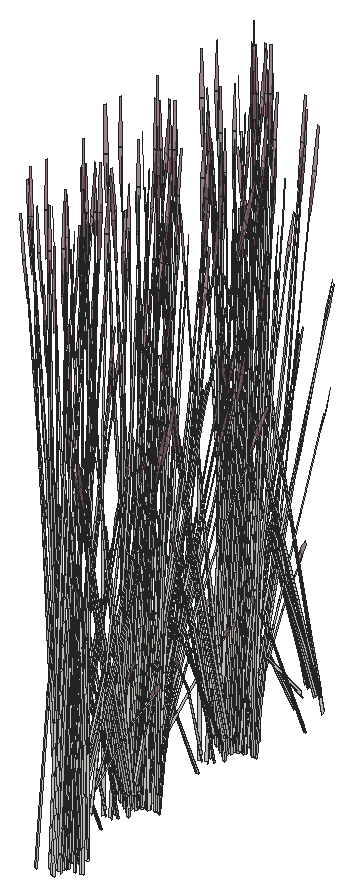
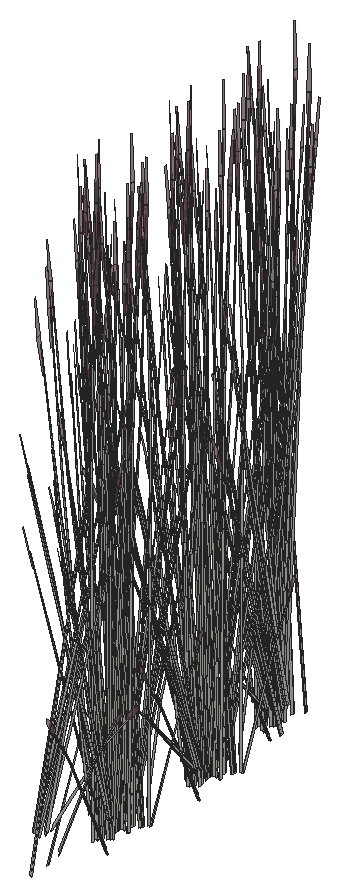
# SketchUp Ruby script. Lengths in inches.
U = 1.inch
M = Sketchup.active_model
def pt(a) = Geom::Point3d.new(a.map { |v| v * U })
def face(e, loops, mat)
  f = e.add_face(loops[0].map { |a| pt(a) })
  loops[1..].each { |l| e.add_face(l.map { |a| pt(a) }).erase! }
  f.material = f.back_material = mat if mat
  f
end
# faces: each face lists its corners as indices into pts; further lists are holes
def faces(e, pts, list, mat = nil) = list.each { |f| face(e, (f[0].is_a?(Array) ? f : [f]).map { |l| l.map { |i| pts[i] } }, mat) }
# xy, xz, yz: faces in a plane at the given z, y or x. An outline is a flat list of corners, or four numbers for a rectangle; further outlines are holes
def ring(l) = l.size == 4 ? [[l[0], l[1]], [l[2], l[1]], [l[2], l[3]], [l[0], l[3]]] : l.each_slice(2).to_a
def flat(e, list, mat, &to3) = list.each { |f| face(e, (f[0].is_a?(Array) ? f : [f]).map { |l| ring(l).map { |u, v| to3.(u, v) } }, mat) }
def xy(e, z, list, mat = nil) = flat(e, list, mat) { |x, y| [x, y, z] }
def xz(e, y, list, mat = nil) = flat(e, list, mat) { |x, z| [x, y, z] }
def yz(e, x, list, mat = nil) = flat(e, list, mat) { |y, z| [x, y, z] }
def lines(e, pts, list) = list.each { |a, b| e.add_line(pt(pts[a]), pt(pts[b])) }
# prism: a flat outline (further loops are holes) pulled along v
def prism(e, loops, v, mat = nil)
  f = face(e, loops, mat); d = Geom::Vector3d.new(v.map { |x| x * U })
  f.pushpull(f.normal.samedirection?(d) ? d.length : -d.length)
end
def box(e, o, s, mat = nil) = prism(e, [[o, [o[0] + s[0], o[1], o[2]], [o[0] + s[0], o[1] + s[1], o[2]], [o[0], o[1] + s[1], o[2]]]], [0, 0, s[2]], mat)
def at(x, y, z, deg = 0) = Geom::Transformation.translation(pt([x, y, z])) * Geom::Transformation.rotation(ORIGIN, Z_AXIS, deg.degrees)
def axes(o, x, y, z) = Geom::Transformation.new([*x, 0, *y, 0, *z, 0, *pt(o).to_a, 1])
def part(name) = M.definitions.add(name)
# library, detail: a bought-in or finely detailed component or shape, given as its bounding box
def library(name, o, s) = part(name).tap { |d| box(d.entities, o, s) }
def detail(e, o, s) = box(e.add_group.entities, o, s)
def put(e, d, t, mat = nil) = e.add_instance(d, t).tap { |i| i.material = mat if mat }
def group(e, t, mat = nil) = e.add_group.tap { |g| g.transformation = t; g.material = mat if mat }.entities
root = M.entities
M.materials.add("LightPink_Translucent").color = [144, 107, 117]
M.materials["LightPink_Translucent"].alpha = 0.75
c1 = part("blade")
p = [[2.15,0.21,22],[0,0.17,0],[0.09,0.45,0],[2.18,0.31,22],[2.29,0.31,22],[0.38,0.45,0],
  [2.48,0.24,33],[2.49,0.24,33],[2.48,0.22,33]]
faces(c1.entities,p,[[0,1,2,3],[4,5,2,3],[6,3,4,7],[8,0,3,6]])
c2 = part("seeds")
p = [[0.3,-0.1,1.38],[-0.01,-0.03,1.59],[-0.01,-0.03,0.03],[0.14,-0.07,-0.07],[0.29,-0.03,3],[0.15,0.01,3.11]]
faces(c2.entities,p,[[0,1,2,3],[1,0,4,5]],"LightPink_Translucent")
c3 = part("blade with seeds")
put(c3.entities,c1,at(0,0,0))
put(c3.entities,c2,axes([2.4,0.25,30.99],[1.5799,-0.05474,1.17369],[-0.12525,1.92788,0.29478],[-0.07173,-0.02425,1.56792]))
put(root,c3,axes([405.15,364.68,-9.95],[0,-0.62892,0],[0.63949,0,0],[0,0,1.6711]))
put(root,c3,axes([404.84,364.29,-9.8],[-0.42403,0.49328,0.42607],[-0.50377,-0.43543,0.16719],[0.10223,-0.04923,1.47927]))
put(root,c3,axes([405.31,365.17,-9.86],[-0.47569,-0.46784,-0.05709],[0.47598,-0.46812,0],[-0.01661,-0.01634,1.63492]))
put(root,c3,axes([404.11,363.47,-9.7],[-0.14774,0.54019,0.16428],[-0.54062,-0.15287,0.32672],[0.09339,-0.00263,1.49371]))
put(root,c3,axes([404.4,365.23,-9.8],[0.64638,0.11452,0.42607],[-0.13155,0.64678,0.16719],[-0.09446,-0.06245,1.47927]))
put(root,c3,axes([404.05,366.26,-9.7],[0.54955,-0.14427,0.16428],[0.1357,0.53689,0.32672],[-0.04901,-0.07823,1.49371]))
put(root,c3,axes([405.74,363.5,-9.7],[-0.54955,0.14427,0.16428],[-0.1357,-0.53689,0.32672],[0.04901,0.07823,1.49371]))
put(root,c3,axes([405.4,364.54,-9.78],[-0.64638,-0.11452,0.45814],[0.13155,-0.64678,0.17978],[0.09446,0.06245,1.59061]))
put(root,c3,axes([404.88,366.13,-9.95],[-0.16686,-0.46861,0],[0.47648,-0.16411,0],[0,0,1.4375]))
put(root,c3,axes([405.69,366.29,-9.7],[0.14774,-0.54019,0.16428],[0.54062,0.15287,0.32672],[-0.09339,0.00263,1.49371]))
put(root,c3,axes([405.57,365.0625,-9.9375],[0.35699,0.35109,0],[-0.35699,0.35109,0],[0,0,1.57621]))
put(root,c3,axes([406.53,364.91,-9.7],[-0.40181,-0.39593,0.16428],[0.40492,-0.38402,0.32672],[-0.04438,0.08086,1.49371]))
put(root,c3,axes([404.76,366.34,-9.95],[-0.51557,-0.24403,0],[0.24813,-0.50705,0],[0,0,1.51513]))
put(root,c3,axes([405.5625,364.65,-9.47],[0.24813,-0.48978,0.41661],[0.51557,0.23571,-0.2005],[0,0.1129,1.33761]))
put(root,c3,axes([405.47,364.93,-9.87],[0,0.62861,-0.05249],[-0.63949,0,0],[0,0.01975,1.67027]))
put(root,c3,axes([405.43,365.33,-9.47],[0.55535,-0.03355,0.41661],[0.05022,0.55698,-0.2005],[-0.09942,0.05645,1.33761]))
put(root,c3,axes([405.35,366.35,-9.95],[0.51557,0.24403,0],[-0.24813,0.50705,0],[0,0,1.62917]))
put(root,c3,axes([405.55,366.89,-9.96],[-0.31576,-0.54657,-0.04789],[0.53494,-0.30375,0.48057],[-0.13182,0.05204,1.52373]))
put(root,c3,axes([405.44,365.57,-9.5625],[0.37783,0.32657,0.13483],[-0.31516,0.36844,-0.38503],[-0.08772,0.04981,1.18024]))
put(root,c3,axes([405.84,366.58,-9.69],[0.47863,-0.27177,0.46235],[0.28609,0.48733,0],[-0.10901,0.0619,1.46668]))
put(root,c3,axes([405.16,366.15,-9.87],[0.22235,0.62444,-0.05599],[-0.63531,0.21881,0],[0.00776,0.02181,1.60327]))
put(root,c3,axes([405.41,366.82,-10.11],[-0.47712,-0.13449,-0.28847],[0.12013,-0.47362,0.28847],[-0.09619,0.05462,1.29413]))
put(root,c3,axes([407,365.33,-9.95],[-0.63917,-0.00435,-0.04634],[0,-0.60749,0.46507],[-0.02009,0.13829,1.47457]))
put(root,c3,axes([405.33,365.45,-9.52],[0.05959,0.62022,-0.27094],[-0.62068,0.0375,-0.46562],[-0.1093,0.08261,1.4872]))
put(root,c3,axes([405.55,365.21,-9.94],[-0.24813,0.48978,-0.41661],[-0.51557,-0.23571,0.2005],[0,0.1129,1.33761]))
put(root,c3,axes([405.57,366.61,-9.83],[0.64025,0.17667,0.2864],[-0.16018,0.63149,-0.33981],[-0.10597,0.07904,1.53541]))
put(root,c3,axes([405.52,367.04,-10.12],[-0.47863,0.27177,-0.46235],[-0.28609,-0.48733,0],[-0.10901,0.0619,1.46668]))
put(root,c3,axes([404.15,373.01,-9.59],[-0.14537,0.11002,1.33163],[-0.43536,-0.19256,-0.28638],[0.0807,-0.23948,0.56934]))
put(root,c3,axes([403.36,366.375,-7.3],[0.34603,-0.28618,0.32977],[0.32756,0.32677,-0.42575],[-0.04984,0.16603,0.81462]))
put(root,c3,axes([405.95,366.96,-9.79],[0.31974,0.54466,0],[-0.53494,0.30375,-0.48057],[-0.12184,0.06918,1.52448]))
put(root,c3,axes([403.07,372.41,-10.61],[-0.08578,0.01958,1.6421],[-0.47437,-0.22044,-0.25086],[0.00796,-0.18387,0.2797]))
put(root,c3,axes([405.68,364.8,-9.35],[-0.01397,-0.51177,1.31553],[0.63227,0.13266,0.557],[-0.14954,0.28003,1.24175]))
put(root,c3,axes([404.5,373.82,-7.36],[0.01331,-0.50278,-0.66157],[0.56035,0.03377,0.07984],[0.05914,-0.213,0.93586]))
put(root,c3,axes([404.33,366.85,-7.3],[0.15418,-0.41799,0.32977],[0.44981,0.12192,-0.42575],[0.04124,0.16829,0.81462]))
put(root,c3,axes([403.53,373.02,-7.78],[0.15418,-0.41799,-0.32977],[0.44981,0.12192,0.42575],[-0.04124,-0.16829,0.81462]))
put(root,c3,axes([405.17,372.65,-7.62],[-0.05194,0.04152,1.65179],[-0.50886,-0.14007,-0.15608],[-0.01842,-0.18118,0.29231]))
put(root,c3,axes([403.62,372.13,-9.42],[0.06561,0.31695,1.06958],[-0.36394,-0.17555,0.78586],[0.03916,-0.16229,0.23558]))
put(root,c3,axes([404.39,373.66,-7.64],[-0.3661,-0.36521,-0.47583],[0.38674,-0.31985,-0.36857],[0.0557,-0.18556,0.91046]))
put(root,c3,axes([404.9375,368.34,-6.74],[0.35341,-0.31182,-0.06041],[0.32382,0.34152,-0.27392],[0.0228,0.09677,0.90349]))
put(root,c3,axes([403.59,373.11,-7.59],[0.50393,0.1421,0.447],[-0.17232,0.46717,0.36857],[-0.03028,-0.18372,0.92496]))
put(root,c3,axes([404.19,367.23,-7.6],[-0.37684,0.18473,0.05988],[-0.18445,-0.33686,0.47138],[0.03639,0.14849,0.71878]))
put(root,c3,axes([404.77,373.85,-7.3125],[-0.56206,-0.02693,-0.11324],[0.01536,-0.50991,-0.62851],[0.03904,-0.19638,0.95501]))
put(root,c3,axes([403.14,366.45,-6.97],[0.56206,0.02693,-0.12569],[-0.01536,0.50991,-0.69765],[-0.03904,0.19638,1.06006]))
put(root,c3,axes([404.73,373.52,-7.78],[0.34603,-0.28618,-0.32977],[0.32756,0.32677,0.42575],[0.04984,-0.16603,0.81462]))
put(root,c3,axes([404.18,367.02,-7.3125],[0.50045,-0.25306,-0.11324],[0.24593,0.44915,-0.62851],[0.06603,0.18927,0.95501]))
put(root,c3,axes([403.72,373.08,-7.6],[0.37684,-0.18473,0.05988],[0.18445,0.33686,0.47138],[-0.03639,-0.14849,0.71878]))
put(root,c3,axes([404.33,367.19,-7.28],[-0.50393,-0.1421,0.49617],[0.17232,-0.46717,0.40911],[0.03028,0.18372,1.0267]))
put(root,c3,axes([404.27,367.12,-10.61],[0.08277,-0.02958,1.6421],[0.49786,0.16279,-0.25086],[0.01456,0.18348,0.2797]))
put(root,c3,axes([403.53,366.65,-7.34],[0.3661,0.36521,-0.52818],[-0.38674,0.31985,-0.40911],[-0.0557,0.18556,1.01061]))
put(root,c3,axes([403.13,367.2,-9.37],[0.46459,-0.09625,0.0606],[0.10681,0.38778,-0.80367],[-0.02945,0.1963,0.72038]))
put(root,c3,axes([404.61,367,-7.64],[0.50273,0.13626,-0.47583],[-0.17232,0.46717,-0.36857],[0.0461,0.18809,0.91046]))
put(root,c3,axes([404.38,367.29,-7.78],[-0.15418,0.41799,-0.32977],[-0.44981,-0.12192,0.42575],[0.04124,0.16829,0.81462]))
put(root,c3,axes([403.94,366.12,-8.39],[-0.01252,-0.20862,1.59586],[0.54251,0.1384,0.12904],[-0.03356,0.2973,0.68222]))
put(root,c3,axes([404.55,373.93,-7.3],[-0.34603,0.28618,0.32977],[-0.32756,-0.32677,-0.42575],[0.04984,-0.16603,0.81462]))
put(root,c3,axes([402.28,373.45,-9.79],[-0.31974,-0.54466,0],[0.53494,-0.30375,-0.48057],[0.12184,-0.06918,1.52448]))
put(root,c3,axes([404.43,366.91,-7.36],[0.24409,0.44196,-0.66157],[-0.50245,0.2463,0.07984],[0.05708,0.21354,0.93586]))
put(root,c3,axes([404.06,368.03,-7.61],[0.06483,0.08753,1.62908],[0.52315,0.03439,-0.25764],[0.05261,0.19303,0.13065]))
put(root,c3,axes([402.71,373.36,-10.12],[0.47863,-0.27177,-0.46235],[0.28609,0.48733,0],[0.10901,-0.0619,1.46668]))
put(root,c3,axes([402.68,375.2,-9.94],[0.24813,-0.48978,-0.41661],[0.51557,0.23571,0.2005],[0,-0.1129,1.33761]))
put(root,c3,axes([402.9,374.95,-9.52],[-0.05959,-0.62022,-0.27094],[0.62068,-0.0375,-0.46562],[0.1093,-0.08261,1.4872]))
put(root,c3,axes([402.82,373.58,-10.11],[0.47712,0.13449,-0.28847],[-0.12013,0.47362,0.28847],[0.09619,-0.05462,1.29413]))
put(root,c3,axes([402.99,375.4375,-9.73],[0.57623,0.26344,0.22409],[-0.27732,0.5474,0.46562],[0,-0.12618,1.49497]))
put(root,c3,axes([402.8,375.07,-9.47],[-0.55535,0.03355,0.41661],[-0.05022,-0.55698,-0.2005],[0.09942,-0.05645,1.33761]))
put(root,c3,axes([402.78,375.27,-9.8],[0.22235,0.6078,0.42607],[-0.63531,0.21135,0.16719],[0.00776,-0.11168,1.47927]))
put(root,c3,axes([403.58,375.32,-9.95],[0,-0.62892,0],[0.63949,0,0],[0,0,1.6711]))
put(root,c3,axes([404.36,373.87,-9.69],[-0.47863,-0.27177,0.46235],[0.28609,-0.48733,0],[0.10901,0.0619,1.46668]))
put(root,c3,axes([403.28,374.93,-9.8],[-0.42403,0.49328,0.42607],[-0.50377,-0.43543,0.16719],[0.10223,-0.04923,1.47927]))
put(root,c3,axes([403.74,375.8125,-9.86],[-0.47569,-0.46784,-0.05709],[0.47598,-0.46812,0],[-0.01661,-0.01634,1.63492]))
put(root,c3,axes([402.54,374.12,-9.7],[-0.14774,0.54019,0.16428],[-0.54062,-0.15287,0.32672],[0.09339,-0.00263,1.49371]))
put(root,c3,axes([403.67,374.72,-9.5625],[0.09866,-0.48509,0.13483],[0.48202,0.0842,-0.38503],[0.08772,0.04981,1.18024]))
put(root,c3,axes([403.46,374.84,-9.47],[-0.30722,-0.45622,0.41661],[0.46535,-0.32126,-0.2005],[0.09942,0.05645,1.33761]))
put(root,c3,axes([404.01,375.46,-9.95],[0.57217,0,0],[0,0.56272,0],[0,0,1.66132]))
put(root,c3,axes([404.18,374.15,-9.7],[-0.54955,0.14427,0.16428],[-0.1357,-0.53689,0.32672],[0.04901,0.07823,1.49371]))
put(root,c3,axes([403.83,375.18,-9.78],[-0.64638,-0.11452,0.45814],[0.13155,-0.64678,0.17978],[0.09446,0.06245,1.59061]))
put(root,c3,axes([403.3125,376.77,-9.95],[-0.16686,-0.46861,0],[0.47648,-0.16411,0],[0,0,1.4375]))
put(root,c3,axes([403.9375,376.71,-9.97],[0.53691,-0.18442,-0.17877],[0.18866,0.53125,0.00007],[0.05927,-0.02038,1.61933]))
put(root,c3,axes([404,375.71,-9.9375],[0.35699,0.35109,0],[-0.35699,0.35109,0],[0,0,1.57621]))
put(root,c3,axes([404.97,375.55,-9.7],[-0.40181,-0.39593,0.16428],[0.40492,-0.38402,0.32672],[-0.04438,0.08086,1.49371]))
put(root,c3,axes([404,375.3,-9.47],[0.24813,-0.48978,0.41661],[0.51557,0.23571,-0.2005],[0,0.1129,1.33761]))
put(root,c3,axes([403.9,375.58,-9.87],[0,0.62861,-0.05249],[-0.63949,0,0],[0,0.01975,1.67027]))
put(root,c3,axes([403.95,375.13,-9.94],[0.30722,0.45622,-0.41661],[-0.46535,0.32126,0.2005],[0.09942,0.05645,1.33761]))
put(root,c3,axes([405.3,375.57,-9.69],[0,-0.54355,0.46235],[0.57217,0,0],[0,0.1238,1.46668]))
put(root,c3,axes([403.87,375.97,-9.47],[0.55535,-0.03355,0.41661],[0.05022,0.55698,-0.2005],[-0.09942,0.05645,1.33761]))
put(root,c3,axes([404.21,375.41,-9.5625],[0.47648,-0.15851,0.13483],[0.16686,0.45265,-0.38503],[0,0.09962,1.18024]))
put(root,c3,axes([403.78,377,-9.95],[0.51557,0.24403,0],[-0.24813,0.50705,0],[0,0,1.62917]))
put(root,c3,axes([404.28,377.22,-9.69],[0.47863,-0.27177,0.46235],[0.28609,0.48733,0],[-0.10901,0.0619,1.46668]))
put(root,c3,axes([403.6,376.79,-9.87],[0.22235,0.62444,-0.05599],[-0.63531,0.21881,0],[0.00776,0.02181,1.60327]))
put(root,c3,axes([405.43,375.97,-9.95],[-0.63917,-0.00435,-0.04634],[0,-0.60749,0.46507],[-0.02009,0.13829,1.47457]))
put(root,c3,axes([404.05,375.44,-9.52],[0.57594,0.25935,-0.27094],[-0.27732,0.5474,-0.46562],[0.0181,0.1344,1.4872]))
put(root,c3,axes([405.3,376.0625,-10.11],[-0.35699,0.33913,-0.28847],[-0.35699,-0.33913,0.28847],[0,0.10923,1.29413]))
put(root,c3,axes([403.99,375.85,-9.94],[-0.24813,0.48978,-0.41661],[-0.51557,-0.23571,0.2005],[0,0.1129,1.33761]))
put(root,c3,axes([403.85,377.42,-7.3],[-0.07899,-0.43781,0.32977],[0.45153,-0.11561,-0.42575],[0.12128,0.12546,0.81462]))
put(root,c3,axes([404,377.26,-9.83],[0.64025,0.17667,0.2864],[-0.16018,0.63149,-0.33981],[-0.10597,0.07904,1.53541]))
put(root,c3,axes([405.54,376.07,-10.12],[0,0.54355,-0.46235],[-0.57217,0,0],[0,0.1238,1.46668]))
put(root,c3,axes([404.15,374.9,-7.83],[-0.44191,-0.28242,1.28769],[0.46662,-0.43971,0.5556],[0.14258,0.26499,1.24467]))
put(root,c3,axes([404.43,383.87,-9.59],[-0.14537,0.11002,1.33163],[-0.43536,-0.19256,-0.28638],[0.0807,-0.23948,0.56934]))
put(root,c3,axes([404.28,376,-10.05],[0.18752,0.49766,-0.6445],[-0.54017,0.17923,-0.16915],[0.02073,0.16852,1.42262]))
put(root,c3,axes([403.35,383.27,-10.61],[-0.08578,0.01958,1.6421],[-0.47437,-0.22044,-0.25086],[0.00796,-0.18387,0.2797]))
put(root,c3,axes([402.77,377.49,-7.3],[0.15418,-0.41799,0.32977],[0.44981,0.12192,-0.42575],[0.04124,0.16829,0.81462]))
put(root,c3,axes([404.78,384.68,-7.36],[0.01331,-0.50278,-0.66157],[0.56035,0.03377,0.07984],[0.05914,-0.213,0.93586]))
put(root,c3,axes([403.8125,383.875,-7.78],[0.15418,-0.41799,-0.32977],[0.44981,0.12192,0.42575],[-0.04124,-0.16829,0.81462]))
put(root,c3,axes([405.45,383.51,-7.62],[-0.05194,0.04152,1.65179],[-0.50886,-0.14007,-0.15608],[-0.01842,-0.18118,0.29231]))
put(root,c3,axes([403.92,377.82,-7.6],[-0.23243,0.34529,0.05988],[-0.331,-0.20103,0.47138],[0.10701,0.1107,0.71878]))
put(root,c3,axes([403.37,378.98,-6.74],[0.35341,-0.31182,-0.06041],[0.32382,0.34152,-0.27392],[0.0228,0.09677,0.90349]))
put(root,c3,axes([404.02,377.72,-7.59],[-0.50866,0.12474,0.447],[-0.08828,-0.48932,0.36857],[0.11963,0.14421,0.92496]))
put(root,c3,axes([403.9,382.99,-9.42],[0.06561,0.31695,1.06958],[-0.36394,-0.17555,0.78586],[0.03916,-0.16229,0.23558]))
put(root,c3,axes([404.67,384.52,-7.64],[-0.3661,-0.36521,-0.47583],[0.38674,-0.31985,-0.36857],[0.0557,-0.18556,0.91046]))
put(root,c3,axes([402.62,377.66,-7.3125],[0.50045,-0.25306,-0.11324],[0.24593,0.44915,-0.62851],[0.06603,0.18927,0.95501]))
put(root,c3,axes([403.87,383.97,-7.59],[0.50393,0.1421,0.447],[-0.17232,0.46717,0.36857],[-0.03028,-0.18372,0.92496]))
put(root,c3,axes([405.05,384.71,-7.3125],[-0.56206,-0.02693,-0.11324],[0.01536,-0.50991,-0.62851],[0.03904,-0.19638,0.95501]))
put(root,c3,axes([404,383.9375,-7.6],[0.37684,-0.18473,0.05988],[0.18445,0.33686,0.47138],[-0.03639,-0.14849,0.71878]))
put(root,c3,axes([402.71,377.76,-10.61],[0.08277,-0.02958,1.6421],[0.49786,0.16279,-0.25086],[0.01456,0.18348,0.2797]))
put(root,c3,axes([403.05,377.64,-7.64],[0.50273,0.13626,-0.47583],[-0.17232,0.46717,-0.36857],[0.0461,0.18809,0.91046]))
put(root,c3,axes([403.33,376.68,-8.39],[-0.1169,-0.17452,1.59586],[0.54019,-0.14692,0.12904],[0.12209,0.27397,0.68222]))
put(root,c3,axes([402.82,377.93,-7.78],[-0.15418,0.41799,-0.32977],[-0.44981,-0.12192,0.42575],[0.04124,0.16829,0.81462]))
put(root,c3,axes([403.86,384.32,-7.3],[-0.15418,0.41799,0.32977],[-0.44981,-0.12192,-0.42575],[-0.04124,-0.16829,0.81462]))
put(root,c3,axes([402.86,377.55,-7.36],[0.24409,0.44196,-0.66157],[-0.50245,0.2463,0.07984],[0.05708,0.21354,0.93586]))
put(root,c3,axes([404.83,384.79,-7.3],[-0.34603,0.28618,0.32977],[-0.32756,-0.32677,-0.42575],[0.04984,-0.16603,0.81462]))
put(root,c3,axes([402.56,384.31,-9.79],[-0.31974,-0.54466,0],[0.53494,-0.30375,-0.48057],[0.12184,-0.06918,1.52448]))
put(root,c3,axes([402.5,378.67,-7.61],[0.06483,0.08753,1.62908],[0.52315,0.03439,-0.25764],[0.05261,0.19303,0.13065]))
put(root,c3,axes([402.99,384.22,-10.12],[0.47863,-0.27177,-0.46235],[0.28609,0.48733,0],[0.10901,-0.0619,1.46668]))
put(root,c3,axes([402.96,386.05,-9.94],[0.24813,-0.48978,-0.41661],[0.51557,0.23571,0.2005],[0,-0.1129,1.33761]))
put(root,c3,axes([403.19,385.8125,-9.52],[-0.05959,-0.62022,-0.27094],[0.62068,-0.0375,-0.46562],[0.1093,-0.08261,1.4872]))
put(root,c3,axes([403.1,384.4375,-10.11],[0.47712,0.13449,-0.28847],[-0.12013,0.47362,0.28847],[0.09619,-0.05462,1.29413]))
put(root,c3,axes([403.27,386.3,-9.73],[0.57623,0.26344,0.22409],[-0.27732,0.5474,0.46562],[0,-0.12618,1.49497]))
put(root,c3,axes([403.08,385.93,-9.47],[-0.55535,0.03355,0.41661],[-0.05022,-0.55698,-0.2005],[0.09942,-0.05645,1.33761]))
put(root,c3,axes([403.0625,386.13,-9.8],[0.22235,0.6078,0.42607],[-0.63531,0.21135,0.16719],[0.00776,-0.11168,1.47927]))
put(root,c3,axes([403.86,386.18,-9.95],[0,-0.62892,0],[0.63949,0,0],[0,0,1.6711]))
put(root,c3,axes([404.64,384.73,-9.69],[-0.47863,-0.27177,0.46235],[0.28609,-0.48733,0],[0.10901,0.0619,1.46668]))
put(root,c3,axes([403.56,385.79,-9.8],[-0.42403,0.49328,0.42607],[-0.50377,-0.43543,0.16719],[0.10223,-0.04923,1.47927]))
put(root,c3,axes([404.02,386.67,-9.86],[-0.47569,-0.46784,-0.05709],[0.47598,-0.46812,0],[-0.01661,-0.01634,1.63492]))
put(root,c3,axes([402.82,384.97,-9.7],[-0.14774,0.54019,0.16428],[-0.54062,-0.15287,0.32672],[0.09339,-0.00263,1.49371]))
put(root,c3,axes([403.95,385.58,-9.5625],[0.09866,-0.48509,0.13483],[0.48202,0.0842,-0.38503],[0.08772,0.04981,1.18024]))
put(root,c3,axes([403.74,385.7,-9.47],[-0.30722,-0.45622,0.41661],[0.46535,-0.32126,-0.2005],[0.09942,0.05645,1.33761]))
put(root,c3,axes([404.29,386.32,-9.95],[0.57217,0,0],[0,0.56272,0],[0,0,1.66132]))
put(root,c3,axes([404.46,385,-9.7],[-0.54955,0.14427,0.16428],[-0.1357,-0.53689,0.32672],[0.04901,0.07823,1.49371]))
put(root,c3,axes([404.11,386.04,-9.78],[-0.64638,-0.11452,0.45814],[0.13155,-0.64678,0.17978],[0.09446,0.06245,1.59061]))
put(root,c3,axes([403.59,387.63,-9.95],[-0.16686,-0.46861,0],[0.47648,-0.16411,0],[0,0,1.4375]))
put(root,c3,axes([404.22,387.57,-9.97],[0.53691,-0.18442,-0.17877],[0.18866,0.53125,0.00007],[0.05927,-0.02038,1.61933]))
put(root,c3,axes([404.4,387.79,-9.7],[0.14774,-0.54019,0.16428],[0.54062,0.15287,0.32672],[-0.09339,0.00263,1.49371]))
put(root,c3,axes([404.28,386.56,-9.9375],[0.35699,0.35109,0],[-0.35699,0.35109,0],[0,0,1.57621]))
put(root,c3,axes([405.25,386.41,-9.7],[-0.40181,-0.39593,0.16428],[0.40492,-0.38402,0.32672],[-0.04438,0.08086,1.49371]))
put(root,c3,axes([403.48,387.85,-9.95],[-0.51557,-0.24403,0],[0.24813,-0.50705,0],[0,0,1.51513]))
put(root,c3,axes([404.28,386.15,-9.47],[0.24813,-0.48978,0.41661],[0.51557,0.23571,-0.2005],[0,0.1129,1.33761]))
put(root,c3,axes([404.18,386.43,-9.87],[0,0.62861,-0.05249],[-0.63949,0,0],[0,0.01975,1.67027]))
put(root,c3,axes([405.58,386.43,-9.69],[0,-0.54355,0.46235],[0.57217,0,0],[0,0.1238,1.46668]))
put(root,c3,axes([404.15,386.83,-9.47],[0.55535,-0.03355,0.41661],[0.05022,0.55698,-0.2005],[-0.09942,0.05645,1.33761]))
put(root,c3,axes([404.49,386.27,-9.5625],[0.47648,-0.15851,0.13483],[0.16686,0.45265,-0.38503],[0,0.09962,1.18024]))
put(root,c3,axes([404.0625,387.86,-9.95],[0.51557,0.24403,0],[-0.24813,0.50705,0],[0,0,1.62917]))
put(root,c3,axes([404.16,387.07,-9.5625],[0.37783,0.32657,0.13483],[-0.31516,0.36844,-0.38503],[-0.08772,0.04981,1.18024]))
put(root,c3,axes([404.56,388.08,-9.69],[0.47863,-0.27177,0.46235],[0.28609,0.48733,0],[-0.10901,0.0619,1.46668]))
put(root,c3,axes([403.875,387.65,-9.87],[0.22235,0.62444,-0.05599],[-0.63531,0.21881,0],[0.00776,0.02181,1.60327]))
put(root,c3,axes([405.71,386.83,-9.95],[-0.63917,-0.00435,-0.04634],[0,-0.60749,0.46507],[-0.02009,0.13829,1.47457]))
put(root,c3,axes([404.33,386.3,-9.52],[0.57594,0.25935,-0.27094],[-0.27732,0.5474,-0.46562],[0.0181,0.1344,1.4872]))
put(root,c3,axes([405.53,392.65,-7.61],[-0.07822,-0.07621,1.62908],[-0.52201,0.04832,-0.25764],[-0.08331,-0.18228,0.13065]))
put(root,c3,axes([405.58,386.92,-10.11],[-0.35699,0.33913,-0.28847],[-0.35699,-0.33913,0.28847],[0,0.10923,1.29413]))
put(root,c3,axes([406.07,393.9375,-7.36],[-0.24409,-0.44196,-0.66157],[0.50245,-0.2463,0.07984],[-0.05708,-0.21354,0.93586]))
put(root,c3,axes([404.27,386.71,-9.94],[-0.24813,0.48978,-0.41661],[-0.51557,-0.23571,0.2005],[0,0.1129,1.33761]))
put(root,c3,axes([405.65,392.96,-10.61],[-0.08578,0.01958,1.6421],[-0.47437,-0.22044,-0.25086],[0.00796,-0.18387,0.2797]))
put(root,c3,axes([404.28,388.11,-9.83],[0.64025,0.17667,0.2864],[-0.16018,0.63149,-0.33981],[-0.10597,0.07904,1.53541]))
put(root,c3,axes([406.12,393.56,-7.78],[0.15418,-0.41799,-0.32977],[0.44981,0.12192,0.42575],[-0.04124,-0.16829,0.81462]))
put(root,c3,axes([405.82,386.93,-10.12],[0,0.54355,-0.46235],[-0.57217,0,0],[0,0.1238,1.46668]))
put(root,c3,axes([405.89,393.85,-7.64],[-0.50273,-0.13626,-0.47583],[0.17232,-0.46717,-0.36857],[-0.0461,-0.18809,0.91046]))
put(root,c3,axes([404.89,393.55,-7.26],[0.56969,-0.13971,0.50064],[0.09887,0.54803,0.4128],[-0.13398,-0.16152,1.03595]))
put(root,c3,axes([404.67,388.46,-9.79],[0.31974,0.54466,0],[-0.53494,0.30375,-0.48057],[-0.12184,0.06918,1.52448]))
put(root,c3,axes([404.56,386.86,-10.05],[0.18752,0.49766,-0.6445],[-0.54017,0.17923,-0.16915],[0.02073,0.16852,1.42262]))
put(root,c3,axes([406.32,393.82,-7.3125],[-0.50045,0.25306,-0.11324],[-0.24593,-0.44915,-0.62851],[-0.06603,-0.18927,0.95501]))
put(root,c3,axes([404.33,393.06,-9.42],[0.26677,0.18918,1.06958],[-0.38851,0.11372,0.78586],[-0.08313,-0.14539,0.23558]))
put(root,c3,axes([403.05,388.35,-7.3],[0.15418,-0.41799,0.32977],[0.44981,0.12192,-0.42575],[0.04124,0.16829,0.81462]))
put(root,c3,axes([404.2,388.68,-7.6],[-0.23243,0.34529,0.05988],[-0.331,-0.20103,0.47138],[0.10701,0.1107,0.71878]))
put(root,c3,axes([403.65,389.84,-6.74],[0.35341,-0.31182,-0.06041],[0.32382,0.34152,-0.27392],[0.0228,0.09677,0.90349]))
put(root,c3,axes([405.02,393.67,-7.6],[0.23243,-0.34529,0.05988],[0.331,0.20103,0.47138],[-0.10701,-0.1107,0.71878]))
put(root,c3,axes([404.3,388.58,-7.59],[-0.50866,0.12474,0.447],[-0.08828,-0.48932,0.36857],[0.11963,0.14421,0.92496]))
put(root,c3,axes([404.94,395.6,-10.05],[-0.21003,-0.55738,-0.65031],[0.60499,-0.20074,-0.17068],[-0.02321,-0.18874,1.43544]))
put(root,c3,axes([406.17,394,-7.3],[-0.15418,0.41799,0.32977],[-0.44981,-0.12192,-0.42575],[-0.04124,-0.16829,0.81462]))
put(root,c3,axes([402.91,388.73,-7.6],[-0.37684,0.18473,0.05988],[-0.18445,-0.33686,0.47138],[0.03639,0.14849,0.71878]))
put(root,c3,axes([402.9,388.52,-7.3125],[0.50045,-0.25306,-0.11324],[0.24593,0.44915,-0.62851],[0.06603,0.18927,0.95501]))
put(root,c3,axes([403.04,388.69,-7.28],[-0.50393,-0.1421,0.49617],[0.17232,-0.46717,0.40911],[0.03028,0.18372,1.0267]))
put(root,c3,axes([402.99,388.62,-10.61],[0.08277,-0.02958,1.6421],[0.49786,0.16279,-0.25086],[0.01456,0.18348,0.2797]))
